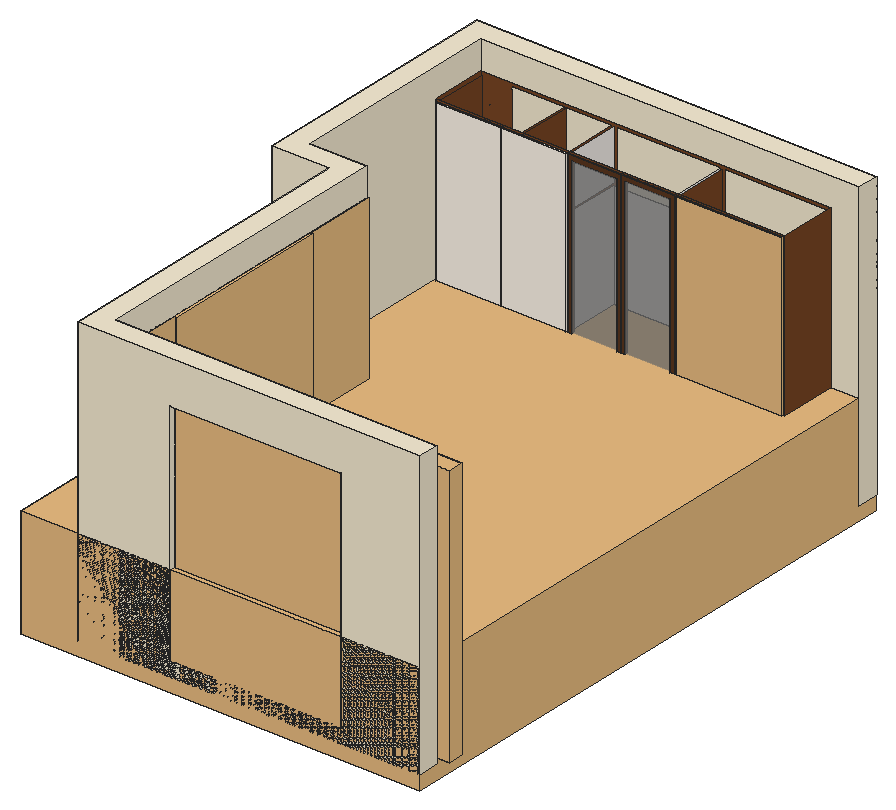
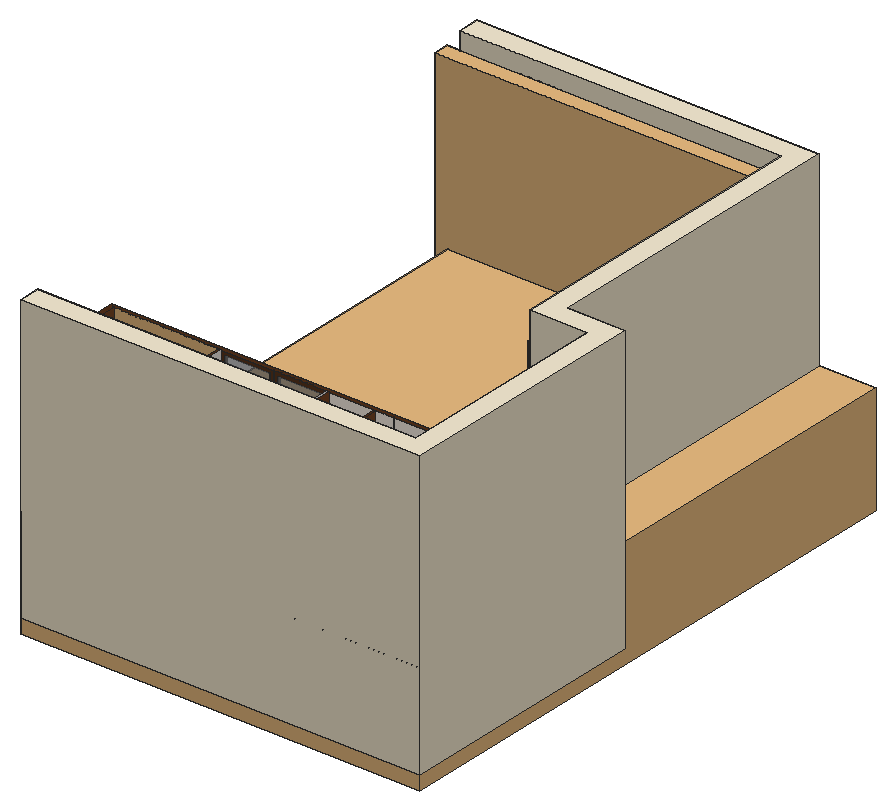
# SketchUp Ruby script. Lengths in inches.
U = 1.inch
M = Sketchup.active_model
def pt(a) = Geom::Point3d.new(a.map { |v| v * U })
def face(e, loops, mat)
  f = e.add_face(loops[0].map { |a| pt(a) })
  loops[1..].each { |l| e.add_face(l.map { |a| pt(a) }).erase! }
  f.material = f.back_material = mat if mat
  f
end
# faces: each face lists its corners as indices into pts; further lists are holes
def faces(e, pts, list, mat = nil) = list.each { |f| face(e, (f[0].is_a?(Array) ? f : [f]).map { |l| l.map { |i| pts[i] } }, mat) }
# xy, xz, yz: faces in a plane at the given z, y or x. An outline is a flat list of corners, or four numbers for a rectangle; further outlines are holes
def ring(l) = l.size == 4 ? [[l[0], l[1]], [l[2], l[1]], [l[2], l[3]], [l[0], l[3]]] : l.each_slice(2).to_a
def flat(e, list, mat, &to3) = list.each { |f| face(e, (f[0].is_a?(Array) ? f : [f]).map { |l| ring(l).map { |u, v| to3.(u, v) } }, mat) }
def xy(e, z, list, mat = nil) = flat(e, list, mat) { |x, y| [x, y, z] }
def xz(e, y, list, mat = nil) = flat(e, list, mat) { |x, z| [x, y, z] }
def yz(e, x, list, mat = nil) = flat(e, list, mat) { |y, z| [x, y, z] }
def lines(e, pts, list) = list.each { |a, b| e.add_line(pt(pts[a]), pt(pts[b])) }
# prism: a flat outline (further loops are holes) pulled along v
def prism(e, loops, v, mat = nil)
  f = face(e, loops, mat); d = Geom::Vector3d.new(v.map { |x| x * U })
  f.pushpull(f.normal.samedirection?(d) ? d.length : -d.length)
end
def box(e, o, s, mat = nil) = prism(e, [[o, [o[0] + s[0], o[1], o[2]], [o[0] + s[0], o[1] + s[1], o[2]], [o[0], o[1] + s[1], o[2]]]], [0, 0, s[2]], mat)
def at(x, y, z, deg = 0) = Geom::Transformation.translation(pt([x, y, z])) * Geom::Transformation.rotation(ORIGIN, Z_AXIS, deg.degrees)
def axes(o, x, y, z) = Geom::Transformation.new([*x, 0, *y, 0, *z, 0, *pt(o).to_a, 1])
def part(name) = M.definitions.add(name)
# library, detail: a bought-in or finely detailed component or shape, given as its bounding box
def library(name, o, s) = part(name).tap { |d| box(d.entities, o, s) }
def detail(e, o, s) = box(e.add_group.entities, o, s)
def put(e, d, t, mat = nil) = e.add_instance(d, t).tap { |i| i.material = mat if mat }
def group(e, t, mat = nil) = e.add_group.tap { |g| g.transformation = t; g.material = mat if mat }.entities
root = M.entities
M.materials.add("0001 AP 9436 AIR BREEZE").color = [243, 237, 232]
M.materials.add("0993 AP 7924 MOON YEAR").color = [247, 236, 211]
M.materials.add("Teddy_Skin").color = [228, 212, 199]
M.materials.add("[Translucent Glass Gray]").color = [128, 128, 128]
M.materials["[Translucent Glass Gray]"].alpha = 0.5
M.materials.add("[Wax 01]").color = [255, 246, 234]
M.materials.add("[Wood Veneer 01]").color = [91, 55, 31]
M.materials.add("[Wood Veneer 01]3").color = [120, 70, 37]
c1 = library("Group\#10",[0,0,-5.36],[198,135,41.44])
c2 = library("1",[0,-0.85,0],[30,0.85,108.17])
c3 = library("Vanity Chair",[-7.875,-7.875,0],[15.75,15.75,16.41])
c4 = library("Group\#4",[0,-1.41,0],[72,1.41,108.17])
c5 = library("Group5_1",[-7.56,-66.38,0.11],[6.33,135.04,120.95])
c6 = library("6",[-5.88,-5.88,-12.16],[13.32,13.32,12.16])
c7 = part("3")
box(c7.entities,[-0.39,0,0],[0.39,19.24,99],"[Translucent Glass Gray]")
c8 = library("Group\#20",[-1,-0.04,0],[1,44.08,102])
c9 = library("sliding door",[152.33,87.51,0.76],[72,5.24,96])
xy(root,6,[[24,0,24,141,33,141,33,9,168,9,168,0],[0,132,0,240,168,240,168,231,156,231,156,213,9,213,9,132],[9,132,24,141]],"0993 AP 7924 MOON YEAR")
xy(root,10,[[9,213,156,231]],"0993 AP 7924 MOON YEAR")
xy(root,10,[[9,207,156,231]],"[Wood Veneer 01]3")
xy(root,11,[[65.5,207,110,230]],"0001 AP 9436 AIR BREEZE")
xy(root,11,[[10,207,64.5,207,64.5,230,45.5,230,45.5,208,44.5,208,44.5,230,10,230],[111,207,155,230],[44.5,208,45.5,208,45.5,230,64,230,64,231,22,231,22,230,44.5,230],[66,230,109.5,231],[111.5,230,155,231]],"[Wood Veneer 01]3")
xy(root,12,[[63,0,135,9]],"0993 AP 7924 MOON YEAR")
xy(root,21.44,[[10,209,44.5,230],[45.5,209,64.5,230]],"[Wood Veneer 01]3")
xy(root,22.44,[[10,209,44.5,230],[45.5,209,64.5,230]],"[Wood Veneer 01]3")
xy(root,22.5,[[[65.5,208,110,230],[87.65,217.5,87.85,217.5,87.89,217.51,88.04,217.54,88.08,217.56,88.13,217.57,88.21,217.61,88.26,217.64,88.3,217.66,88.34,217.69,88.41,217.75,88.45,217.78,88.51,217.86,88.54,217.89,88.6,217.97,88.625,218.01,88.67,218.1,88.69,218.15,88.7,218.19,88.71,218.24,88.73,218.28,88.74,218.33,88.74,218.38,88.75,218.43,88.75,218.57,88.74,218.62,88.74,218.67,88.73,218.72,88.71,218.76,88.7,218.81,88.69,218.85,88.67,218.9,88.625,218.99,88.6,219.03,88.54,219.11,88.51,219.14,88.45,219.22,88.41,219.25,88.34,219.31,88.3,219.34,88.26,219.36,88.21,219.39,88.13,219.43,88.08,219.44,88.04,219.46,87.89,219.49,87.85,219.5,87.65,219.5,87.61,219.49,87.46,219.46,87.42,219.44,87.37,219.43,87.29,219.39,87.24,219.36,87.2,219.34,87.16,219.31,87.09,219.25,87.05,219.22,86.99,219.14,86.96,219.11,86.9,219.03,86.875,218.99,86.83,218.9,86.81,218.85,86.8,218.81,86.79,218.76,86.77,218.72,86.76,218.67,86.76,218.62,86.75,218.57,86.75,218.43,86.76,218.38,86.76,218.33,86.77,218.28,86.79,218.24,86.8,218.19,86.81,218.15,86.83,218.1,86.875,218.01,86.9,217.97,86.96,217.89,86.99,217.86,87.05,217.78,87.09,217.75,87.16,217.69,87.2,217.66,87.24,217.64,87.29,217.61,87.37,217.57,87.42,217.56,87.46,217.54,87.61,217.51]]],"0001 AP 9436 AIR BREEZE")
xy(root,22.5,[[111,208,155,230]],"[Wood Veneer 01]3")
xy(root,23,[[87.65,217.5,87.61,217.51,87.46,217.54,87.42,217.56,87.37,217.57,87.29,217.61,87.24,217.64,87.2,217.66,87.16,217.69,87.09,217.75,87.05,217.78,86.99,217.86,86.96,217.89,86.9,217.97,86.875,218.01,86.83,218.1,86.81,218.15,86.8,218.19,86.79,218.24,86.77,218.28,86.76,218.33,86.76,218.38,86.75,218.43,86.75,218.57,86.76,218.62,86.76,218.67,86.77,218.72,86.79,218.76,86.8,218.81,86.81,218.85,86.83,218.9,86.875,218.99,86.9,219.03,86.96,219.11,86.99,219.14,87.05,219.22,87.09,219.25,87.16,219.31,87.2,219.34,87.24,219.36,87.29,219.39,87.37,219.43,87.42,219.44,87.46,219.46,87.61,219.49,87.65,219.5,87.85,219.5,87.89,219.49,88.04,219.46,88.08,219.44,88.13,219.43,88.21,219.39,88.26,219.36,88.3,219.34,88.34,219.31,88.41,219.25,88.45,219.22,88.51,219.14,88.54,219.11,88.6,219.03,88.625,218.99,88.67,218.9,88.69,218.85,88.7,218.81,88.71,218.76,88.73,218.72,88.74,218.67,88.74,218.62,88.75,218.57,88.75,218.43,88.74,218.38,88.74,218.33,88.73,218.28,88.71,218.24,88.7,218.19,88.69,218.15,88.67,218.1,88.625,218.01,88.6,217.97,88.54,217.89,88.51,217.86,88.45,217.78,88.41,217.75,88.34,217.69,88.3,217.66,88.26,217.64,88.21,217.61,88.13,217.57,88.08,217.56,88.04,217.54,87.89,217.51,87.85,217.5]],"0001 AP 9436 AIR BREEZE")
xy(root,23.5,[[65.5,208,110,230]],"0001 AP 9436 AIR BREEZE")
xy(root,23.5,[[111,208,155,230]],"[Wood Veneer 01]3")
xy(root,34,[[10,209,44.5,230],[45.5,209,64.5,230]],"[Wood Veneer 01]3")
xy(root,35,[[[65.5,208,110,230],[87.65,217.5,87.85,217.5,87.89,217.51,88.04,217.54,88.08,217.56,88.13,217.57,88.21,217.61,88.26,217.64,88.3,217.66,88.34,217.69,88.41,217.75,88.45,217.78,88.51,217.86,88.54,217.89,88.6,217.97,88.625,218.01,88.67,218.1,88.69,218.15,88.7,218.19,88.71,218.24,88.73,218.28,88.74,218.33,88.74,218.38,88.75,218.43,88.75,218.57,88.74,218.62,88.74,218.67,88.73,218.72,88.71,218.76,88.7,218.81,88.69,218.85,88.67,218.9,88.625,218.99,88.6,219.03,88.54,219.11,88.51,219.14,88.45,219.22,88.41,219.25,88.34,219.31,88.3,219.34,88.26,219.36,88.21,219.39,88.13,219.43,88.08,219.44,88.04,219.46,87.89,219.49,87.85,219.5,87.65,219.5,87.61,219.49,87.46,219.46,87.42,219.44,87.37,219.43,87.29,219.39,87.24,219.36,87.2,219.34,87.16,219.31,87.09,219.25,87.05,219.22,86.99,219.14,86.96,219.11,86.9,219.03,86.875,218.99,86.83,218.9,86.81,218.85,86.8,218.81,86.79,218.76,86.77,218.72,86.76,218.67,86.76,218.62,86.75,218.57,86.75,218.43,86.76,218.38,86.76,218.33,86.77,218.28,86.79,218.24,86.8,218.19,86.81,218.15,86.83,218.1,86.875,218.01,86.9,217.97,86.96,217.89,86.99,217.86,87.05,217.78,87.09,217.75,87.16,217.69,87.2,217.66,87.24,217.64,87.29,217.61,87.37,217.57,87.42,217.56,87.46,217.54,87.61,217.51]]],"0001 AP 9436 AIR BREEZE")
xy(root,35,[[111,208,155,230],[10,209,44.5,230],[45.5,209,64.5,230]],"[Wood Veneer 01]3")
xy(root,35.5,[[87.65,217.5,87.61,217.51,87.46,217.54,87.42,217.56,87.37,217.57,87.29,217.61,87.24,217.64,87.2,217.66,87.16,217.69,87.09,217.75,87.05,217.78,86.99,217.86,86.96,217.89,86.9,217.97,86.875,218.01,86.83,218.1,86.81,218.15,86.8,218.19,86.79,218.24,86.77,218.28,86.76,218.33,86.76,218.38,86.75,218.43,86.75,218.57,86.76,218.62,86.76,218.67,86.77,218.72,86.79,218.76,86.8,218.81,86.81,218.85,86.83,218.9,86.875,218.99,86.9,219.03,86.96,219.11,86.99,219.14,87.05,219.22,87.09,219.25,87.16,219.31,87.2,219.34,87.24,219.36,87.29,219.39,87.37,219.43,87.42,219.44,87.46,219.46,87.61,219.49,87.65,219.5,87.85,219.5,87.89,219.49,88.04,219.46,88.08,219.44,88.13,219.43,88.21,219.39,88.26,219.36,88.3,219.34,88.34,219.31,88.41,219.25,88.45,219.22,88.51,219.14,88.54,219.11,88.6,219.03,88.625,218.99,88.67,218.9,88.69,218.85,88.7,218.81,88.71,218.76,88.73,218.72,88.74,218.67,88.74,218.62,88.75,218.57,88.75,218.43,88.74,218.38,88.74,218.33,88.73,218.28,88.71,218.24,88.7,218.19,88.69,218.15,88.67,218.1,88.625,218.01,88.6,217.97,88.54,217.89,88.51,217.86,88.45,217.78,88.41,217.75,88.34,217.69,88.3,217.66,88.26,217.64,88.21,217.61,88.13,217.57,88.08,217.56,88.04,217.54,87.89,217.51,87.85,217.5]],"0001 AP 9436 AIR BREEZE")
xy(root,36,[[65.5,208,110,230]],"0001 AP 9436 AIR BREEZE")
xy(root,36,[[111,208,155,230]],"[Wood Veneer 01]3")
xy(root,108,[[63,0,135,9]],"0993 AP 7924 MOON YEAR")
xy(root,126,[[24,0,168,0,168,9,33,9,33,141,9,141,9,231,168,231,168,240,0,240,0,132,24,132]],"0993 AP 7924 MOON YEAR")
xz(root,0,[[[24,6,168,126],[63,12,135,108]]],"0993 AP 7924 MOON YEAR")
xz(root,9,[[[33,6,168,126],[63,12,135,108]]],"0993 AP 7924 MOON YEAR")
xz(root,132,[[0,6,24,126]],"0993 AP 7924 MOON YEAR")
xz(root,141,[[9,6,33,126]],"0993 AP 7924 MOON YEAR")
xz(root,207,[[[9,10,156,114],[10,11,64.5,113],[65.5,11,110,113],[111,11,155,113]]],"[Wood Veneer 01]3")
xz(root,208,[[65.5,22.5,110,23.5],[65.5,35,110,36]],"0001 AP 9436 AIR BREEZE")
xz(root,208,[[44.5,11,45.5,113],[111,22.5,155,23.5],[111,35,155,36]],"[Wood Veneer 01]3")
xz(root,209,[[10,21.44,44.5,22.44],[45.5,21.44,64.5,22.44],[10,34,44.5,35],[45.5,34,64.5,35]],"[Wood Veneer 01]3")
xz(root,213,[[9,6,156,10]],"0993 AP 7924 MOON YEAR")
xz(root,217.5,[[87.65,22.5,87.7,23],[87.7,22.5,87.75,23],[87.75,22.5,87.8,23],[87.8,22.5,87.85,23],[87.65,35,87.7,35.5],
  [87.7,35,87.75,35.5],[87.75,35,87.8,35.5],[87.8,35,87.85,35.5]],"0001 AP 9436 AIR BREEZE")
xz(root,219.5,[[87.65,22.5,87.7,23],[87.7,22.5,87.75,23],[87.75,22.5,87.8,23],[87.8,22.5,87.85,23],[87.65,35,87.7,35.5],
  [87.7,35,87.75,35.5],[87.75,35,87.8,35.5],[87.8,35,87.85,35.5]],"0001 AP 9436 AIR BREEZE")
xz(root,230,[[65.5,11,110,22.5],[65.5,23.5,110,35],[65.5,36,110,91]],"0001 AP 9436 AIR BREEZE")
xz(root,230,[[10,11,44.5,21.44],[45.5,11,64.5,21.44],[111,11,155,22.5],[10,22.44,44.5,34],[45.5,22.44,64.5,34],
  [111,23.5,155,35],[10,35,44.5,90.94],[45.5,35,64.5,90.94],[111,36,155,91]],"[Wood Veneer 01]3")
xz(root,231,[[156,6,168,6,168,126,9,126,9,10,156,10]],"0993 AP 7924 MOON YEAR")
xz(root,231,[[[9,10,156,114],[111.5,11,155,113],[66,11,109.5,113],[22,11,64,113]]],"[Wood Veneer 01]3")
xz(root,240,[[0,6,168,126]],"0993 AP 7924 MOON YEAR")
yz(root,0,[[132,6,240,126]],"0993 AP 7924 MOON YEAR")
yz(root,9,[[141,6,213,6,213,10,231,10,231,126,141,126]],"0993 AP 7924 MOON YEAR")
yz(root,9,[[207,10,231,114]],"[Wood Veneer 01]3")
yz(root,10,[[207,11,230,11,230,21.44,209,21.44,209,22.44,230,22.44,230,34,209,34,209,35,230,35,230,90.94,209,90.94,209,91.94,230,91.94,230,113,207,113]],"[Wood Veneer 01]3")
yz(root,24,[[0,6,132,126]],"0993 AP 7924 MOON YEAR")
yz(root,33,[[9,6,141,126]],"0993 AP 7924 MOON YEAR")
yz(root,44.5,[[208,11,208,113,230,113,230,91.94,209,91.94,209,90.94,230,90.94,230,35,209,35,209,34,230,34,230,22.44,209,22.44,209,21.44,230,21.44,230,11]],"[Wood Veneer 01]3")
yz(root,45.5,[[208,11,230,11,230,21.44,209,21.44,209,22.44,230,22.44,230,34,209,34,209,35,230,35,230,90.94,209,90.94,209,91.94,230,91.94,230,113,208,113]],"[Wood Veneer 01]3")
yz(root,63,[[0,12,9,108]],"0993 AP 7924 MOON YEAR")
yz(root,64.5,[[207,11,207,113,230,113,230,91.94,209,91.94,209,90.94,230,90.94,230,35,209,35,209,34,230,34,230,22.44,209,22.44,209,21.44,230,21.44,230,11]],"[Wood Veneer 01]3")
yz(root,65.5,[[207,11,230,11,230,22.5,208,22.5,208,23.5,230,23.5,230,35,208,35,208,36,230,36,230,91,208,91,208,92,230,92,230,113,207,113]],"0001 AP 9436 AIR BREEZE")
yz(root,86.75,[[218.43,22.5,218.48,23],[218.48,22.5,218.52,23],[218.52,22.5,218.57,23],[218.43,35,218.48,35.5],[218.48,35,218.52,35.5],
  [218.52,35,218.57,35.5]],"0001 AP 9436 AIR BREEZE")
yz(root,86.76,[[218.33,22.5,218.38,23],[218.62,22.5,218.67,23],[218.33,35,218.38,35.5],[218.62,35,218.67,35.5]],"0001 AP 9436 AIR BREEZE")
yz(root,88.74,[[218.33,22.5,218.38,23],[218.62,22.5,218.67,23],[218.33,35,218.38,35.5],[218.62,35,218.67,35.5]],"0001 AP 9436 AIR BREEZE")
yz(root,88.75,[[218.43,22.5,218.48,23],[218.48,22.5,218.52,23],[218.52,22.5,218.57,23],[218.43,35,218.48,35.5],[218.48,35,218.52,35.5],
  [218.52,35,218.57,35.5]],"0001 AP 9436 AIR BREEZE")
yz(root,110,[[207,11,207,113,230,113,230,92,208,92,208,91,230,91,230,36,208,36,208,35,230,35,230,23.5,208,23.5,208,22.5,230,22.5,230,11]],"0001 AP 9436 AIR BREEZE")
yz(root,111,[[207,11,230,11,230,22.5,208,22.5,208,23.5,230,23.5,230,35,208,35,208,36,230,36,230,91,208,91,208,92,230,92,230,113,207,113]],"[Wood Veneer 01]3")
yz(root,135,[[0,12,9,108]],"0993 AP 7924 MOON YEAR")
yz(root,155,[[207,11,207,113,230,113,230,92,208,92,208,91,230,91,230,36,208,36,208,35,230,35,230,23.5,208,23.5,208,22.5,230,22.5,230,11],[230,11,230,22.5,208,22.5,208,23.5,230,23.5,230,35,208,35,208,36,230,36,230,91,208,91,208,92,230,92,230,113,231,113,231,11]],"[Wood Veneer 01]3")
yz(root,156,[[213,6,231,10]],"0993 AP 7924 MOON YEAR")
yz(root,156,[[207,10,231,114]],"[Wood Veneer 01]3")
yz(root,168,[[0,6,9,126],[231,6,240,126]],"0993 AP 7924 MOON YEAR")
p = [[87.46,217.54,22.5],[87.42,217.56,22.5],[87.42,217.56,23],[87.46,217.54,23],[87.56,217.52,22.5],[87.51,217.53,22.5],
  [87.51,217.53,23],[87.56,217.52,23],[87.65,217.5,22.5],[87.61,217.51,22.5],[87.61,217.51,23],[87.65,217.5,23],
  [87.89,217.51,22.5],[87.85,217.5,22.5],[87.85,217.5,23],[87.89,217.51,23],[87.99,217.53,22.5],[87.94,217.52,22.5],
  [87.94,217.52,23],[87.99,217.53,23],[88.08,217.56,22.5],[88.04,217.54,22.5],[88.04,217.54,23],[88.08,217.56,23],
  [87.29,217.61,22.5],[87.24,217.64,22.5],[87.24,217.64,23],[87.29,217.61,23],[87.2,217.66,22.5],[87.2,217.66,23],
  [87.37,217.57,22.5],[87.33,217.59,22.5],[87.33,217.59,23],[87.37,217.57,23],[88.17,217.59,22.5],[88.13,217.57,22.5],
  [88.13,217.57,23],[88.17,217.59,23],[88.26,217.64,22.5],[88.21,217.61,22.5],[88.21,217.61,23],[88.26,217.64,23],
  [88.3,217.66,22.5],[88.3,217.66,23],[87.16,217.69,22.5],[87.125,217.72,22.5],[87.125,217.72,23],[87.16,217.69,23],
  [87.09,217.75,22.5],[87.09,217.75,23],[88.375,217.72,22.5],[88.34,217.69,22.5],[88.34,217.69,23],[88.375,217.72,23],
  [88.41,217.75,22.5],[88.41,217.75,23],[87.05,217.78,22.5],[87.02,217.82,22.5],[87.02,217.82,23],[87.05,217.78,23],
  [86.99,217.86,22.5],[86.99,217.86,23],[88.48,217.82,22.5],[88.45,217.78,22.5],[88.45,217.78,23],[88.48,217.82,23],
  [88.51,217.86,22.5],[88.51,217.86,23],[86.96,217.89,22.5],[86.93,217.93,22.5],[86.93,217.93,23],[86.96,217.89,23],
  [86.9,217.97,22.5],[86.9,217.97,23],[88.57,217.93,22.5],[88.54,217.89,22.5],[88.54,217.89,23],[88.57,217.93,23],
  [88.6,217.97,22.5],[88.6,217.97,23],[86.875,218.01,22.5],[86.875,218.01,23],[86.85,218.06,22.5],[86.85,218.06,23],
  [88.65,218.06,22.5],[88.625,218.01,22.5],[88.625,218.01,23],[88.65,218.06,23],[86.83,218.1,22.5],[86.83,218.1,23],
  [86.81,218.15,22.5],[86.81,218.15,23],[86.8,218.19,22.5],[86.8,218.19,23],[88.67,218.1,22.5],[88.67,218.1,23],
  [88.7,218.19,22.5],[88.69,218.15,22.5],[88.69,218.15,23],[88.7,218.19,23],[86.79,218.24,22.5],[86.79,218.24,23],
  [86.77,218.28,22.5],[86.77,218.28,23],[88.73,218.28,22.5],[88.71,218.24,22.5],[88.71,218.24,23],[88.73,218.28,23],
  [86.76,218.33,22.5],[86.76,218.33,23],[88.74,218.33,22.5],[88.74,218.33,23],[86.76,218.38,22.5],[86.75,218.43,22.5],
  [86.75,218.43,23],[86.76,218.38,23],[88.75,218.43,22.5],[88.74,218.38,22.5],[88.74,218.38,23],[88.75,218.43,23],
  [86.75,218.57,22.5],[86.76,218.62,22.5],[86.76,218.62,23],[86.75,218.57,23],[88.74,218.62,22.5],[88.75,218.57,22.5],
  [88.75,218.57,23],[88.74,218.62,23],[86.76,218.67,22.5],[86.77,218.72,22.5],[86.77,218.72,23],[86.76,218.67,23],
  [86.79,218.76,22.5],[86.79,218.76,23],[88.71,218.76,22.5],[88.73,218.72,22.5],[88.73,218.72,23],[88.71,218.76,23],
  [88.74,218.67,22.5],[88.74,218.67,23],[86.8,218.81,22.5],[86.8,218.81,23],[86.81,218.85,22.5],[86.81,218.85,23],
  [88.69,218.85,22.5],[88.7,218.81,22.5],[88.7,218.81,23],[88.69,218.85,23],[86.83,218.9,22.5],[86.83,218.9,23],
  [86.85,218.94,22.5],[86.85,218.94,23],[86.875,218.99,22.5],[86.875,218.99,23],[88.625,218.99,22.5],[88.65,218.94,22.5],
  [88.65,218.94,23],[88.625,218.99,23],[88.67,218.9,22.5],[88.67,218.9,23],[86.9,219.03,22.5],[86.9,219.03,23],
  [86.93,219.07,22.5],[86.93,219.07,23],[88.57,219.07,22.5],[88.6,219.03,22.5],[88.6,219.03,23],[88.57,219.07,23],
  [86.96,219.11,22.5],[86.96,219.11,23],[86.99,219.14,22.5],[86.99,219.14,23],[87.02,219.18,22.5],[87.02,219.18,23],
  [88.48,219.18,22.5],[88.51,219.14,22.5],[88.51,219.14,23],[88.48,219.18,23],[88.54,219.11,22.5],[88.54,219.11,23],
  [87.05,219.22,22.5],[87.05,219.22,23],[87.09,219.25,22.5],[87.09,219.25,23],[87.125,219.28,22.5],[87.125,219.28,23],
  [88.375,219.28,22.5],[88.41,219.25,22.5],[88.41,219.25,23],[88.375,219.28,23],[88.45,219.22,22.5],[88.45,219.22,23],
  [87.16,219.31,22.5],[87.16,219.31,23],[87.2,219.34,22.5],[87.2,219.34,23],[87.24,219.36,22.5],[87.24,219.36,23],
  [88.26,219.36,22.5],[88.3,219.34,22.5],[88.3,219.34,23],[88.26,219.36,23],[88.34,219.31,22.5],[88.34,219.31,23],
  [87.29,219.39,22.5],[87.29,219.39,23],[87.33,219.41,22.5],[87.33,219.41,23],[87.37,219.43,22.5],[87.37,219.43,23],
  [87.42,219.44,22.5],[87.42,219.44,23],[87.46,219.46,22.5],[87.46,219.46,23],[88.04,219.46,22.5],[88.08,219.44,22.5],
  [88.08,219.44,23],[88.04,219.46,23],[88.13,219.43,22.5],[88.13,219.43,23],[88.17,219.41,22.5],[88.17,219.41,23],
  [88.21,219.39,22.5],[88.21,219.39,23],[87.51,219.47,22.5],[87.51,219.47,23],[87.56,219.48,22.5],[87.56,219.48,23],
  [87.61,219.49,22.5],[87.61,219.49,23],[87.65,219.5,22.5],[87.65,219.5,23],[87.85,219.5,22.5],[87.89,219.49,22.5],
  [87.89,219.49,23],[87.85,219.5,23],[87.94,219.48,22.5],[87.94,219.48,23],[87.99,219.47,22.5],[87.99,219.47,23],
  [87.46,217.54,35],[87.42,217.56,35],[87.42,217.56,35.5],[87.46,217.54,35.5],[87.56,217.52,35],[87.51,217.53,35],
  [87.51,217.53,35.5],[87.56,217.52,35.5],[87.65,217.5,35],[87.61,217.51,35],[87.61,217.51,35.5],[87.65,217.5,35.5],
  [87.89,217.51,35],[87.85,217.5,35],[87.85,217.5,35.5],[87.89,217.51,35.5],[87.99,217.53,35],[87.94,217.52,35],
  [87.94,217.52,35.5],[87.99,217.53,35.5],[88.08,217.56,35],[88.04,217.54,35],[88.04,217.54,35.5],[88.08,217.56,35.5],
  [87.29,217.61,35],[87.24,217.64,35],[87.24,217.64,35.5],[87.29,217.61,35.5],[87.2,217.66,35],[87.2,217.66,35.5],
  [87.37,217.57,35],[87.33,217.59,35],[87.33,217.59,35.5],[87.37,217.57,35.5],[88.17,217.59,35],[88.13,217.57,35],
  [88.13,217.57,35.5],[88.17,217.59,35.5],[88.26,217.64,35],[88.21,217.61,35],[88.21,217.61,35.5],[88.26,217.64,35.5],
  [88.3,217.66,35],[88.3,217.66,35.5],[87.16,217.69,35],[87.125,217.72,35],[87.125,217.72,35.5],[87.16,217.69,35.5],
  [87.09,217.75,35],[87.09,217.75,35.5],[88.375,217.72,35],[88.34,217.69,35],[88.34,217.69,35.5],[88.375,217.72,35.5],
  [88.41,217.75,35],[88.41,217.75,35.5],[87.05,217.78,35],[87.02,217.82,35],[87.02,217.82,35.5],[87.05,217.78,35.5],
  [86.99,217.86,35],[86.99,217.86,35.5],[88.48,217.82,35],[88.45,217.78,35],[88.45,217.78,35.5],[88.48,217.82,35.5],
  [88.51,217.86,35],[88.51,217.86,35.5],[86.96,217.89,35],[86.93,217.93,35],[86.93,217.93,35.5],[86.96,217.89,35.5],
  [86.9,217.97,35],[86.9,217.97,35.5],[88.57,217.93,35],[88.54,217.89,35],[88.54,217.89,35.5],[88.57,217.93,35.5],
  [88.6,217.97,35],[88.6,217.97,35.5],[86.875,218.01,35],[86.875,218.01,35.5],[86.85,218.06,35],[86.85,218.06,35.5],
  [88.65,218.06,35],[88.625,218.01,35],[88.625,218.01,35.5],[88.65,218.06,35.5],[86.83,218.1,35],[86.83,218.1,35.5],
  [86.81,218.15,35],[86.81,218.15,35.5],[86.8,218.19,35],[86.8,218.19,35.5],[88.67,218.1,35],[88.67,218.1,35.5],
  [88.7,218.19,35],[88.69,218.15,35],[88.69,218.15,35.5],[88.7,218.19,35.5],[86.79,218.24,35],[86.79,218.24,35.5],
  [86.77,218.28,35],[86.77,218.28,35.5],[88.73,218.28,35],[88.71,218.24,35],[88.71,218.24,35.5],[88.73,218.28,35.5],
  [86.76,218.33,35],[86.76,218.33,35.5],[88.74,218.33,35],[88.74,218.33,35.5],[86.76,218.38,35],[86.75,218.43,35],
  [86.75,218.43,35.5],[86.76,218.38,35.5],[88.75,218.43,35],[88.74,218.38,35],[88.74,218.38,35.5],[88.75,218.43,35.5],
  [86.75,218.57,35],[86.76,218.62,35],[86.76,218.62,35.5],[86.75,218.57,35.5],[88.74,218.62,35],[88.75,218.57,35],
  [88.75,218.57,35.5],[88.74,218.62,35.5],[86.76,218.67,35],[86.77,218.72,35],[86.77,218.72,35.5],[86.76,218.67,35.5],
  [86.79,218.76,35],[86.79,218.76,35.5],[88.71,218.76,35],[88.73,218.72,35],[88.73,218.72,35.5],[88.71,218.76,35.5],
  [88.74,218.67,35],[88.74,218.67,35.5],[86.8,218.81,35],[86.8,218.81,35.5],[86.81,218.85,35],[86.81,218.85,35.5],
  [88.69,218.85,35],[88.7,218.81,35],[88.7,218.81,35.5],[88.69,218.85,35.5],[86.83,218.9,35],[86.83,218.9,35.5],
  [86.85,218.94,35],[86.85,218.94,35.5],[86.875,218.99,35],[86.875,218.99,35.5],[88.625,218.99,35],[88.65,218.94,35],
  [88.65,218.94,35.5],[88.625,218.99,35.5],[88.67,218.9,35],[88.67,218.9,35.5],[86.9,219.03,35],[86.9,219.03,35.5],
  [86.93,219.07,35],[86.93,219.07,35.5],[88.57,219.07,35],[88.6,219.03,35],[88.6,219.03,35.5],[88.57,219.07,35.5],
  [86.96,219.11,35],[86.96,219.11,35.5],[86.99,219.14,35],[86.99,219.14,35.5],[87.02,219.18,35],[87.02,219.18,35.5],
  [88.48,219.18,35],[88.51,219.14,35],[88.51,219.14,35.5],[88.48,219.18,35.5],[88.54,219.11,35],[88.54,219.11,35.5],
  [87.05,219.22,35],[87.05,219.22,35.5],[87.09,219.25,35],[87.09,219.25,35.5],[87.125,219.28,35],[87.125,219.28,35.5],
  [88.375,219.28,35],[88.41,219.25,35],[88.41,219.25,35.5],[88.375,219.28,35.5],[88.45,219.22,35],[88.45,219.22,35.5],
  [87.16,219.31,35],[87.16,219.31,35.5],[87.2,219.34,35],[87.2,219.34,35.5],[87.24,219.36,35],[87.24,219.36,35.5],
  [88.26,219.36,35],[88.3,219.34,35],[88.3,219.34,35.5],[88.26,219.36,35.5],[88.34,219.31,35],[88.34,219.31,35.5],
  [87.29,219.39,35],[87.29,219.39,35.5],[87.33,219.41,35],[87.33,219.41,35.5],[87.37,219.43,35],[87.37,219.43,35.5],
  [87.42,219.44,35],[87.42,219.44,35.5],[87.46,219.46,35],[87.46,219.46,35.5],[88.04,219.46,35],[88.08,219.44,35],
  [88.08,219.44,35.5],[88.04,219.46,35.5],[88.13,219.43,35],[88.13,219.43,35.5],[88.17,219.41,35],[88.17,219.41,35.5],
  [88.21,219.39,35],[88.21,219.39,35.5],[87.51,219.47,35],[87.51,219.47,35.5],[87.56,219.48,35],[87.56,219.48,35.5],
  [87.61,219.49,35],[87.61,219.49,35.5],[87.65,219.5,35],[87.65,219.5,35.5],[87.85,219.5,35],[87.89,219.49,35],
  [87.89,219.49,35.5],[87.85,219.5,35.5],[87.94,219.48,35],[87.94,219.48,35.5],[87.99,219.47,35],[87.99,219.47,35.5]]
faces(root,p,[[0,1,2,3],[4,5,6,7],[5,0,3,6],[8,9,10,11],[9,4,7,10],[12,13,14,15],[16,17,18,19],[17,12,15,18],
  [20,21,22,23],[21,16,19,22],[24,25,26,27],[25,28,29,26],[30,31,32,33],[31,24,27,32],[1,30,33,2],[34,35,36,37],
  [35,20,23,36],[38,39,40,41],[39,34,37,40],[42,38,41,43],[44,45,46,47],[45,48,49,46],[28,44,47,29],[50,51,52,53],
  [51,42,43,52],[54,50,53,55],[56,57,58,59],[57,60,61,58],[48,56,59,49],[62,63,64,65],[63,54,55,64],[66,62,65,67],
  [68,69,70,71],[69,72,73,70],[60,68,71,61],[74,75,76,77],[75,66,67,76],[78,74,77,79],[72,80,81,73],[80,82,83,81],
  [84,85,86,87],[85,78,79,86],[82,88,89,83],[88,90,91,89],[90,92,93,91],[94,84,87,95],[96,97,98,99],[97,94,95,98],
  [92,100,101,93],[100,102,103,101],[104,105,106,107],[105,96,99,106],[102,108,109,103],[110,104,107,111],[112,113,114,115],[116,117,118,119],
  [120,121,122,123],[124,125,126,127],[128,129,130,131],[129,132,133,130],[134,135,136,137],[135,138,139,136],[132,140,141,133],[140,142,143,141],
  [144,145,146,147],[145,134,137,146],[142,148,149,143],[148,150,151,149],[150,152,153,151],[154,155,156,157],[155,158,159,156],[158,144,147,159],
  [152,160,161,153],[160,162,163,161],[164,165,166,167],[165,154,157,166],[162,168,169,163],[168,170,171,169],[170,172,173,171],[174,175,176,177],
  [175,178,179,176],[178,164,167,179],[172,180,181,173],[180,182,183,181],[182,184,185,183],[186,187,188,189],[187,190,191,188],[190,174,177,191],
  [184,192,193,185],[192,194,195,193],[194,196,197,195],[198,199,200,201],[199,202,203,200],[202,186,189,203],[196,204,205,197],[204,206,207,205],
  [206,208,209,207],[208,210,211,209],[210,212,213,211],[214,215,216,217],[215,218,219,216],[218,220,221,219],[220,222,223,221],[222,198,201,223],
  [212,224,225,213],[224,226,227,225],[226,228,229,227],[228,230,231,229],[232,233,234,235],[233,236,237,234],[236,238,239,237],[238,214,217,239],
  [240,241,242,243],[244,245,246,247],[245,240,243,246],[248,249,250,251],[249,244,247,250],[252,253,254,255],[256,257,258,259],[257,252,255,258],
  [260,261,262,263],[261,256,259,262],[264,265,266,267],[265,268,269,266],[270,271,272,273],[271,264,267,272],[241,270,273,242],[274,275,276,277],
  [275,260,263,276],[278,279,280,281],[279,274,277,280],[282,278,281,283],[284,285,286,287],[285,288,289,286],[268,284,287,269],[290,291,292,293],
  [291,282,283,292],[294,290,293,295],[296,297,298,299],[297,300,301,298],[288,296,299,289],[302,303,304,305],[303,294,295,304],[306,302,305,307],
  [308,309,310,311],[309,312,313,310],[300,308,311,301],[314,315,316,317],[315,306,307,316],[318,314,317,319],[312,320,321,313],[320,322,323,321],
  [324,325,326,327],[325,318,319,326],[322,328,329,323],[328,330,331,329],[330,332,333,331],[334,324,327,335],[336,337,338,339],[337,334,335,338],
  [332,340,341,333],[340,342,343,341],[344,345,346,347],[345,336,339,346],[342,348,349,343],[350,344,347,351],[352,353,354,355],[356,357,358,359],
  [360,361,362,363],[364,365,366,367],[368,369,370,371],[369,372,373,370],[374,375,376,377],[375,378,379,376],[372,380,381,373],[380,382,383,381],
  [384,385,386,387],[385,374,377,386],[382,388,389,383],[388,390,391,389],[390,392,393,391],[394,395,396,397],[395,398,399,396],[398,384,387,399],
  [392,400,401,393],[400,402,403,401],[404,405,406,407],[405,394,397,406],[402,408,409,403],[408,410,411,409],[410,412,413,411],[414,415,416,417],
  [415,418,419,416],[418,404,407,419],[412,420,421,413],[420,422,423,421],[422,424,425,423],[426,427,428,429],[427,430,431,428],[430,414,417,431],
  [424,432,433,425],[432,434,435,433],[434,436,437,435],[438,439,440,441],[439,442,443,440],[442,426,429,443],[436,444,445,437],[444,446,447,445],
  [446,448,449,447],[448,450,451,449],[450,452,453,451],[454,455,456,457],[455,458,459,456],[458,460,461,459],[460,462,463,461],[462,438,441,463],
  [452,464,465,453],[464,466,467,465],[466,468,469,467],[468,470,471,469],[472,473,474,475],[473,476,477,474],[476,478,479,477],[478,454,457,479]],"0001 AP 9436 AIR BREEZE")
put(root,c1,axes([168,0,6],[0,1.21212,0],[-1.24444,0,0],[0,0,1.12]))
put(root,c2,at(33,9,6,90),"Teddy_Skin")
put(root,c2,at(33,111,6,90),"Teddy_Skin")
put(root,c3,axes([31.16,173.4,6],[0,1.13,0],[-1.13,0,0],[0,0,1.13]))
put(root,c4,at(33,39,6,90))
put(root,c5,axes([106.99,16.56,8.42],[0,1,0],[-1,0,0],[0,0,0.91]))
put(root,c6,at(88.53,217.72,22.9,90),"[Wood Veneer 01]3")
g1 = group(root,at(64.43,207,11),"0001 AP 9436 AIR BREEZE")
xy(g1,-0.25,[[-54.36,-1,-27.19,0],[-27.17,-1,0.32,0]],"[Wax 01]")
xy(g1,37,[[-54.68,-1,-54.36,0]],"[Wax 01]")
xy(g1,102.25,[[-54.68,-1,-27.19,0],[-27.17,-1,0.32,0]],"[Wax 01]")
xz(g1,-1,[[-54.36,-0.25,-27.19,-0.25,-27.19,102.25,-54.68,102.25,-54.68,37,-54.36,37],[-27.17,-0.25,0.32,102.25]],"[Wax 01]")
xz(g1,0,[[-54.36,-0.25,-27.19,37],[-27.17,-0.25,0.32,102.25],[-27.19,0,-27.17,102],[-54.68,37,-27.19,102.25]],"[Wax 01]")
yz(g1,-54.68,[[-1,37,0,102.25]],"[Wax 01]")
yz(g1,-54.36,[[-1,-0.25,0,37]],"[Wax 01]")
yz(g1,-27.19,[[-1,-0.25,0,37],[-1,37,0,102.25]],"[Wax 01]")
yz(g1,-27.17,[[-1,-0.25,0,102.25]],"[Wax 01]")
yz(g1,0.32,[[-1,-0.25,0,102.25]],"[Wax 01]")
p = [[-27.19,-1,37],[-27.17,-1,37]]
lines(g1,p,[[0,1]])
g2 = group(root,at(110,207,11,90),"[Wood Veneer 01]")
xy(g2,-0.25,[[-1,-0.25,0,22.24],[-1,22.26,0,44.75]])
xy(g2,1.5,[[-1,1.5,0,20.74],[-1,23.76,0,43]])
xy(g2,100.5,[[-1,1.5,0,20.74],[-1,23.76,0,43]])
xy(g2,102.25,[[-1,-0.25,0,22.24],[-1,22.26,0,44.75]])
xz(g2,-0.25,[[-1,-0.25,0,102.25]])
xz(g2,1.5,[[-1,1.5,0,100.5]])
xz(g2,20.74,[[-1,1.5,0,100.5]])
xz(g2,22.24,[[-1,-0.25,0,102.25]])
xz(g2,22.26,[[-1,-0.25,0,102.25]])
xz(g2,23.76,[[-1,1.5,0,100.5]])
xz(g2,43,[[-1,1.5,0,100.5]])
xz(g2,44.75,[[-1,-0.25,0,102.25]])
yz(g2,-1,[[[-0.25,-0.25,22.24,102.25],[1.5,1.5,20.74,100.5]],[[22.26,-0.25,44.75,102.25],[23.76,1.5,43,100.5]]])
yz(g2,0,[[[-0.25,-0.25,22.24,102.25],[1.5,1.5,20.74,100.5]],[[22.26,-0.25,44.75,102.25],[23.76,1.5,43,100.5]]])
p = [[0,22.26,0],[0,22.24,0]]
lines(g2,p,[[0,1]])
put(g2,c7,at(-0.3,1.5,1.5))
put(g2,c7,at(-0.3,23.76,1.5))
put(root,c8,axes([155.21,207,10.75],[0,1,0],[-1.00946,0,0],[0,0,1.0049]),"0001 AP 9436 AIR BREEZE")
put(root,c9,at(-89.33,-85.25,11.24))
put(root,c6,at(88.53,217.72,35.4,90),"[Wood Veneer 01]3")
